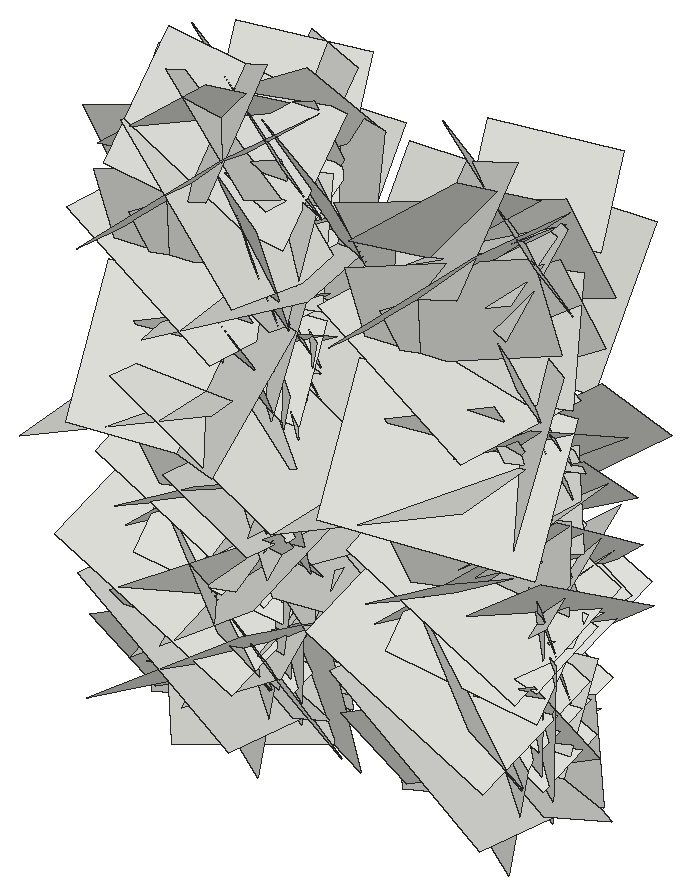
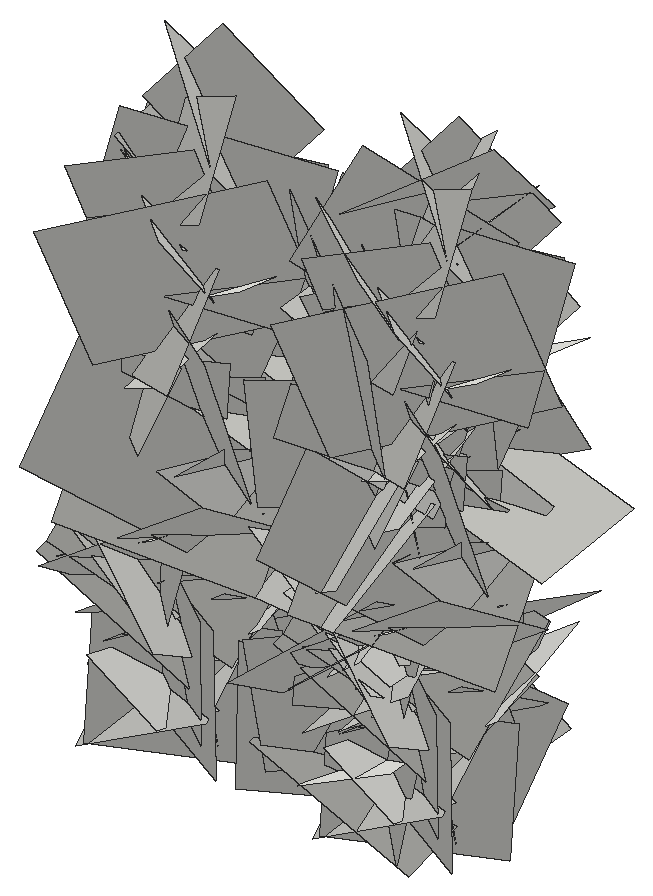
# SketchUp Ruby script. Lengths in inches.
U = 1.inch
M = Sketchup.active_model
def pt(a) = Geom::Point3d.new(a.map { |v| v * U })
def face(e, loops, mat)
  f = e.add_face(loops[0].map { |a| pt(a) })
  loops[1..].each { |l| e.add_face(l.map { |a| pt(a) }).erase! }
  f.material = f.back_material = mat if mat
  f
end
# faces: each face lists its corners as indices into pts; further lists are holes
def faces(e, pts, list, mat = nil) = list.each { |f| face(e, (f[0].is_a?(Array) ? f : [f]).map { |l| l.map { |i| pts[i] } }, mat) }
# xy, xz, yz: faces in a plane at the given z, y or x. An outline is a flat list of corners, or four numbers for a rectangle; further outlines are holes
def ring(l) = l.size == 4 ? [[l[0], l[1]], [l[2], l[1]], [l[2], l[3]], [l[0], l[3]]] : l.each_slice(2).to_a
def flat(e, list, mat, &to3) = list.each { |f| face(e, (f[0].is_a?(Array) ? f : [f]).map { |l| ring(l).map { |u, v| to3.(u, v) } }, mat) }
def xy(e, z, list, mat = nil) = flat(e, list, mat) { |x, y| [x, y, z] }
def xz(e, y, list, mat = nil) = flat(e, list, mat) { |x, z| [x, y, z] }
def yz(e, x, list, mat = nil) = flat(e, list, mat) { |y, z| [x, y, z] }
def lines(e, pts, list) = list.each { |a, b| e.add_line(pt(pts[a]), pt(pts[b])) }
# prism: a flat outline (further loops are holes) pulled along v
def prism(e, loops, v, mat = nil)
  f = face(e, loops, mat); d = Geom::Vector3d.new(v.map { |x| x * U })
  f.pushpull(f.normal.samedirection?(d) ? d.length : -d.length)
end
def box(e, o, s, mat = nil) = prism(e, [[o, [o[0] + s[0], o[1], o[2]], [o[0] + s[0], o[1] + s[1], o[2]], [o[0], o[1] + s[1], o[2]]]], [0, 0, s[2]], mat)
def at(x, y, z, deg = 0) = Geom::Transformation.translation(pt([x, y, z])) * Geom::Transformation.rotation(ORIGIN, Z_AXIS, deg.degrees)
def axes(o, x, y, z) = Geom::Transformation.new([*x, 0, *y, 0, *z, 0, *pt(o).to_a, 1])
def part(name) = M.definitions.add(name)
# library, detail: a bought-in or finely detailed component or shape, given as its bounding box
def library(name, o, s) = part(name).tap { |d| box(d.entities, o, s) }
def detail(e, o, s) = box(e.add_group.entities, o, s)
def put(e, d, t, mat = nil) = e.add_instance(d, t).tap { |i| i.material = mat if mat }
def group(e, t, mat = nil) = e.add_group.tap { |g| g.transformation = t; g.material = mat if mat }.entities
root = M.entities
c1 = part("Component\#6")
p = [[0.01,0,0],[0,3.24,4.54],[4.32,3.24,4.54],[4.33,0,0]]
faces(c1.entities,p,[[0,1,2,3]])
put(root,c1,axes([400.91,170.45,6.95],[-0.13562,-0.59571,0.16409],[0.06684,0.15411,0.60864],[0.65155,-0.13981,-0.02828]))
put(root,c1,axes([404.88,170.45,6.95],[0.13562,-0.59571,0.16409],[-0.06684,0.15411,0.60864],[-0.65155,-0.13981,-0.02828]))
put(root,c1,axes([410.71,170.45,6.95],[-0.13562,-0.59571,0.16409],[0.06684,0.15411,0.60864],[0.65155,-0.13981,-0.02828]))
put(root,c1,axes([404.88,172.51,13.7],[0.18405,-0.71312,-0.93832],[0.0125,-0.94735,0.72216],[-1.2492,-0.11455,-0.13102]))
put(root,c1,axes([400.91,172.51,13.7],[-0.18405,-0.71312,-0.93832],[-0.0125,-0.94735,0.72216],[1.2492,-0.11455,-0.13102]))
put(root,c1,axes([414.68,172.51,13.7],[0.18405,-0.71312,-0.93832],[0.0125,-0.94735,0.72216],[-1.2492,-0.11455,-0.13102]))
put(root,c1,axes([404.88,166.89,12.83],[-0.13197,1.26874,-0.04114],[-0.28106,-0.06642,-1.24587],[-1.31589,-0.11305,0.27023]))
put(root,c1,axes([400.91,166.89,12.83],[0.13197,1.26874,-0.04114],[0.28106,-0.06642,-1.24587],[1.31589,-0.11305,0.27023]))
put(root,c1,axes([414.68,166.89,12.83],[-0.13197,1.26874,-0.04114],[-0.28106,-0.06642,-1.24587],[-1.31589,-0.11305,0.27023]))
put(root,c1,axes([400.91,170.4375,18.81],[-0.19883,-0.70321,0.38228],[-0.06935,0.40479,0.71252],[0.84558,-0.13215,0.14832]))
put(root,c1,axes([404.88,170.4375,18.81],[0.19883,-0.70321,0.38228],[0.06935,0.40479,0.71252],[-0.84558,-0.13215,0.14832]))
put(root,c1,axes([410.71,170.4375,18.81],[-0.19883,-0.70321,0.38228],[-0.06935,0.40479,0.71252],[0.84558,-0.13215,0.14832]))
put(root,c1,axes([404.88,172.01,0.23],[0.18306,-1.21621,0.26629],[0.00588,0.26959,1.22768],[-1.31971,-0.16751,0.04241]))
put(root,c1,axes([400.91,172.01,0.23],[-0.18306,-1.21621,0.26629],[-0.00588,0.26959,1.22768],[1.31971,-0.16751,0.04241]))
put(root,c1,axes([414.68,172.01,0.23],[0.18306,-1.21621,0.26629],[0.00588,0.26959,1.22768],[-1.31971,-0.16751,0.04241]))
put(root,c1,axes([404.88,167.43,21.54],[-0.05686,1.16606,-0.16138],[0.18622,-0.15181,-1.15529],[-1.23383,-0.07665,-0.16693]))
put(root,c1,axes([400.91,167.43,21.54],[0.05686,1.16606,-0.16138],[-0.18622,-0.15181,-1.15529],[1.23383,-0.07665,-0.16693]))
put(root,c1,axes([414.68,167.43,21.54],[-0.05686,1.16606,-0.16138],[0.18622,-0.15181,-1.15529],[-1.23383,-0.07665,-0.16693]))
put(root,c1,axes([404.88,170.29,20.28],[-0.01759,0.35165,-0.94572],[-0.09141,-0.94289,-0.34909],[-1.06561,0.07508,0.04555]))
put(root,c1,axes([400.91,170.29,20.28],[0.01759,0.35165,-0.94572],[0.09141,-0.94289,-0.34909],[1.06561,0.07508,0.04555]))
put(root,c1,axes([414.68,170.29,20.28],[-0.01759,0.35165,-0.94572],[-0.09141,-0.94289,-0.34909],[-1.06561,0.07508,0.04555]))
put(root,c1,axes([404.88,166.61,20.4],[-0.01588,0.7114,0.79833],[0.18087,0.78977,-0.70057],[-1.11894,0.11757,-0.12458]))
put(root,c1,axes([400.91,166.61,20.4],[0.01588,0.7114,0.79833],[-0.18087,0.78977,-0.70057],[1.11894,0.11757,-0.12458]))
put(root,c1,axes([414.68,166.61,20.4],[-0.01588,0.7114,0.79833],[0.18087,0.78977,-0.70057],[-1.11894,0.11757,-0.12458]))
put(root,c1,axes([400.91,169.875,11.58],[-0.08121,-0.31714,0.54408],[0.11401,0.53345,0.32609],[0.65774,-0.13162,0.01065]))
put(root,c1,axes([404.88,169.875,11.58],[0.08121,-0.31714,0.54408],[-0.11401,0.53345,0.32609],[-0.65774,-0.13162,0.01065]))
put(root,c1,axes([410.71,169.875,11.58],[-0.08121,-0.31714,0.54408],[0.11401,0.53345,0.32609],[0.65774,-0.13162,0.01065]))
put(root,c1,axes([404.88,169.82,1.95],[0.02915,-0.64251,0.76006],[0.08177,0.75943,0.6392],[-1.05178,0.04123,0.07076]))
put(root,c1,axes([400.91,169.82,1.95],[-0.02915,-0.64251,0.76006],[-0.08177,0.75943,0.6392],[1.05178,0.04123,0.07076]))
put(root,c1,axes([414.68,169.82,1.95],[0.02915,-0.64251,0.76006],[0.08177,0.75943,0.6392],[-1.05178,0.04123,0.07076]))
put(root,c1,axes([404.88,173.1,4.27],[-0.006,-1.20261,-0.38975],[0.07836,-0.3894,1.20046],[-1.33775,-0.01742,0.07206]))
put(root,c1,axes([400.91,173.1,4.27],[0.006,-1.20261,-0.38975],[-0.07836,-0.3894,1.20046],[1.33775,-0.01742,0.07206]))
put(root,c1,axes([414.68,173.1,4.27],[-0.006,-1.20261,-0.38975],[0.07836,-0.3894,1.20046],[-1.33775,-0.01742,0.07206]))
put(root,c1,axes([400.91,169.57,7.53],[0.02893,-0.34038,0.60393],[-0.06424,0.60091,0.34142],[0.73203,0.06619,0.00609]))
put(root,c1,axes([404.88,169.57,7.53],[-0.02893,-0.34038,0.60393],[0.06424,0.60091,0.34142],[-0.73203,0.06619,0.00609]))
put(root,c1,axes([410.71,169.57,7.53],[0.02893,-0.34038,0.60393],[-0.06424,0.60091,0.34142],[0.73203,0.06619,0.00609]))
put(root,c1,axes([404.88,172.68,14.25],[-0.15371,-1.16437,-0.05617],[-0.14183,-0.0396,1.1664],[-1.22751,0.15038,-0.12774]))
put(root,c1,axes([400.91,172.68,14.25],[0.15371,-1.16437,-0.05617],[0.14183,-0.0396,1.1664],[1.22751,0.15038,-0.12774]))
put(root,c1,axes([414.68,172.68,14.25],[-0.15371,-1.16437,-0.05617],[-0.14183,-0.0396,1.1664],[-1.22751,0.15038,-0.12774]))
put(root,c1,axes([404.88,172.08,18.68],[0.05145,-0.65016,0.07549],[-0.09383,0.06848,0.64671],[-0.68743,-0.05801,-0.08262]))
put(root,c1,axes([400.91,172.08,18.68],[-0.05145,-0.65016,0.07549],[0.09383,0.06848,0.64671],[0.68743,-0.05801,-0.08262]))
put(root,c1,axes([410.71,172.08,18.68],[-0.05145,-0.65016,0.07549],[0.09383,0.06848,0.64671],[0.68743,-0.05801,-0.08262]))
put(root,c1,axes([400.91,168.08,6.15],[-0.10311,0.69666,0.5447],[-0.01855,0.54636,-0.70191],[0.9372,0.08746,0.04604]))
put(root,c1,axes([404.88,168.08,6.15],[0.10311,0.69666,0.5447],[0.01855,0.54636,-0.70191],[-0.9372,0.08746,0.04604]))
put(root,c1,axes([410.71,168.08,6.15],[-0.10311,0.69666,0.5447],[-0.01855,0.54636,-0.70191],[0.9372,0.08746,0.04604]))
put(root,c1,axes([404.88,170.37,5.28],[0.04044,0.69271,-0.86885],[-0.14808,-0.85947,-0.69137],[-1.16852,0.13289,0.05755]))
put(root,c1,axes([400.91,170.37,5.28],[-0.04044,0.69271,-0.86885],[0.14808,-0.85947,-0.69137],[1.16852,0.13289,0.05755]))
put(root,c1,axes([414.68,170.37,5.28],[0.04044,0.69271,-0.86885],[-0.14808,-0.85947,-0.69137],[-1.16852,0.13289,0.05755]))
put(root,c1,axes([404.88,171.61,19.65],[0.05512,0.44879,-0.89687],[0.12411,-0.89465,-0.44089],[-1.05579,-0.08174,-0.09865]))
put(root,c1,axes([400.91,171.61,19.65],[-0.05512,0.44879,-0.89687],[-0.12411,-0.89465,-0.44089],[1.05579,-0.08174,-0.09865]))
put(root,c1,axes([414.68,171.61,19.65],[0.05512,0.44879,-0.89687],[0.12411,-0.89465,-0.44089],[-1.05579,-0.08174,-0.09865]))
put(root,c1,axes([404.88,172.8125,18.6875],[0.10377,-0.25363,-0.96814],[-0.17625,-0.96337,0.23557],[-1.04612,0.13715,-0.13572]))
put(root,c1,axes([400.91,172.8125,18.6875],[-0.10377,-0.25363,-0.96814],[0.17625,-0.96337,0.23557],[1.04612,0.13715,-0.13572]))
put(root,c1,axes([414.68,172.8125,18.6875],[0.10377,-0.25363,-0.96814],[-0.17625,-0.96337,0.23557],[-1.04612,0.13715,-0.13572]))
put(root,c1,axes([404.88,173.43,2.26],[-0.13173,-0.86629,-0.47025],[0.00519,-0.47451,0.87284],[-1.04483,0.10686,0.06363]))
put(root,c1,axes([400.91,173.43,2.26],[0.13173,-0.86629,-0.47025],[-0.00519,-0.47451,0.87284],[1.04483,0.10686,0.06363]))
put(root,c1,axes([414.68,173.43,2.26],[-0.13173,-0.86629,-0.47025],[0.00519,-0.47451,0.87284],[-1.04483,0.10686,0.06363]))
put(root,c1,axes([400.91,172.62,2.82],[-0.11022,-0.07985,-0.84847],[0.01268,-0.85481,0.07898],[0.90326,0.00226,-0.10464]))
put(root,c1,axes([404.88,172.62,2.82],[0.11022,-0.07985,-0.84847],[-0.01268,-0.85481,0.07898],[-0.90326,0.00226,-0.10464]))
put(root,c1,axes([410.71,172.62,2.82],[-0.11022,-0.07985,-0.84847],[0.01268,-0.85481,0.07898],[0.90326,0.00226,-0.10464]))
put(root,c1,axes([404.88,172.18,10.26],[-0.13568,0.14362,-0.9313],[-0.0793,-0.93844,-0.13444],[-0.9957,0.05517,0.13761]))
put(root,c1,axes([414.68,172.18,10.26],[-0.13568,0.14362,-0.9313],[-0.0793,-0.93844,-0.13444],[-0.9957,0.05517,0.13761]))
put(root,c1,axes([400.91,172.18,10.26],[0.13568,0.14362,-0.9313],[0.0793,-0.93844,-0.13444],[0.9957,0.05517,0.13761]))
put(root,c1,axes([400.91,169.25,3.37],[-0.12984,0.58451,0.34416],[-0.01188,0.34794,-0.59491],[0.71891,0.11132,0.05233]))
put(root,c1,axes([404.88,169.25,3.37],[0.12984,0.58451,0.34416],[0.01188,0.34794,-0.59491],[-0.71891,0.11132,0.05233]))
put(root,c1,axes([410.71,169.25,3.37],[-0.12984,0.58451,0.34416],[-0.01188,0.34794,-0.59491],[0.71891,0.11132,0.05233]))
put(root,c1,axes([404.88,174.625,6.88],[-0.07025,-1.10898,-0.49527],[0.16839,-0.49966,1.09755],[-1.27636,-0.00489,0.17206]))
put(root,c1,axes([400.91,174.625,6.88],[0.07025,-1.10898,-0.49527],[-0.16839,-0.49966,1.09755],[1.27636,-0.00489,0.17206]))
put(root,c1,axes([414.68,174.625,6.88],[-0.07025,-1.10898,-0.49527],[0.16839,-0.49966,1.09755],[-1.27636,-0.00489,0.17206]))
put(root,c1,axes([404.88,173.47,4.9],[-0.07332,-0.2848,-0.87141],[0.0336,-0.87411,0.28317],[-0.9712,-0.00874,0.07558]))
put(root,c1,axes([400.91,173.47,4.9],[0.07332,-0.2848,-0.87141],[-0.0336,-0.87411,0.28317],[0.9712,-0.00874,0.07558]))
put(root,c1,axes([414.68,173.47,4.9],[-0.07332,-0.2848,-0.87141],[0.0336,-0.87411,0.28317],[-0.9712,-0.00874,0.07558]))
put(root,c1,axes([400.91,169.67,8.54],[-0.12628,0.08221,0.86907],[-0.11161,0.86937,-0.09667],[0.91857,0.11693,0.10773]))
put(root,c1,axes([404.88,169.67,8.54],[0.12628,0.08221,0.86907],[0.11161,0.86937,-0.09667],[-0.91857,0.11693,0.10773]))
put(root,c1,axes([410.71,169.67,8.54],[-0.12628,0.08221,0.86907],[-0.11161,0.86937,-0.09667],[0.91857,0.11693,0.10773]))
put(root,c1,axes([400.91,173.61,18.42],[0.00387,-0.64214,-0.38262],[0.01033,-0.38255,0.64212],[0.79227,0.00812,-0.0065]))
put(root,c1,axes([404.88,173.61,18.42],[-0.00387,-0.64214,-0.38262],[-0.01033,-0.38255,0.64212],[-0.79227,0.00812,-0.0065]))
put(root,c1,axes([410.71,173.61,18.42],[0.00387,-0.64214,-0.38262],[0.01033,-0.38255,0.64212],[0.79227,0.00812,-0.0065]))
put(root,c1,axes([404.88,173.47,6.03],[0.02519,-0.71274,-0.22366],[-0.1783,-0.22314,0.69319],[-0.7715,0.02829,-0.1675]))
put(root,c1,axes([400.91,173.47,6.03],[-0.02519,-0.71274,-0.22366],[0.1783,-0.22314,0.69319],[0.7715,0.02829,-0.1675]))
put(root,c1,axes([414.68,173.47,6.03],[0.02519,-0.71274,-0.22366],[-0.1783,-0.22314,0.69319],[-0.7715,0.02829,-0.1675]))
put(root,c1,axes([404.88,170.23,14.27],[0.02775,1.05616,-0.50439],[0.01222,-0.50473,-1.05626],[-1.24058,0.01865,-0.02169]))
put(root,c1,axes([400.91,170.23,14.27],[-0.02775,1.05616,-0.50439],[-0.01222,-0.50473,-1.05626],[1.24058,0.01865,-0.02169]))
put(root,c1,axes([414.68,170.23,14.27],[0.02775,1.05616,-0.50439],[0.01222,-0.50473,-1.05626],[-1.24058,0.01865,-0.02169]))
put(root,c1,axes([404.88,172.3,17.31],[0.17712,-0.66279,0.75583],[-0.05377,0.75967,0.67737],[-1.06423,-0.14869,0.09157]))
put(root,c1,axes([400.91,172.3,17.31],[-0.17712,-0.66279,0.75583],[0.05377,0.75967,0.67737],[1.06423,-0.14869,0.09157]))
put(root,c1,axes([414.68,172.3,17.31],[0.17712,-0.66279,0.75583],[-0.05377,0.75967,0.67737],[-1.06423,-0.14869,0.09157]))
put(root,c1,axes([404.88,171.9,21.66],[-0.05821,0.63814,-1.10333],[-0.23209,-1.09266,-0.62107],[-1.33097,0.16262,0.15656]))
put(root,c1,axes([400.91,171.9,21.66],[0.05821,0.63814,-1.10333],[0.23209,-1.09266,-0.62107],[1.33097,0.16262,0.15656]))
put(root,c1,axes([414.68,171.9,21.66],[-0.05821,0.63814,-1.10333],[-0.23209,-1.09266,-0.62107],[-1.33097,0.16262,0.15656]))
put(root,c1,axes([400.91,171.64,6.09],[-0.04085,-0.22846,0.61977],[0.06336,0.61707,0.23119],[0.6973,-0.06945,0.0153]))
put(root,c1,axes([404.88,171.64,6.09],[0.04085,-0.22846,0.61977],[-0.06336,0.61707,0.23119],[-0.6973,-0.06945,0.0153]))
put(root,c1,axes([410.71,171.64,6.09],[-0.04085,-0.22846,0.61977],[0.06336,0.61707,0.23119],[0.6973,-0.06945,0.0153]))
put(root,c1,axes([404.88,170.14,10.52],[-0.06349,0.95893,0.01002],[0.03302,0.01198,-0.96028],[-1.01599,-0.05954,-0.03183]))
put(root,c1,axes([400.91,170.14,10.52],[0.06349,0.95893,0.01002],[-0.03302,0.01198,-0.96028],[1.01599,-0.05954,-0.03183]))
put(root,c1,axes([414.68,170.14,10.52],[-0.06349,0.95893,0.01002],[0.03302,0.01198,-0.96028],[-1.01599,-0.05954,-0.03183]))
put(root,c1,axes([400.91,174.87,19.3],[-0.1513,-0.51657,-0.73784],[-0.06675,-0.7395,0.52991],[0.9524,-0.13389,-0.08008]))
put(root,c1,axes([404.88,174.87,19.3],[0.1513,-0.51657,-0.73784],[0.06675,-0.7395,0.52991],[-0.9524,-0.13389,-0.08008]))
put(root,c1,axes([410.71,174.87,19.3],[-0.1513,-0.51657,-0.73784],[-0.06675,-0.7395,0.52991],[0.9524,-0.13389,-0.08008]))
put(root,c1,axes([404.88,172.92,11.6],[-0.15777,-0.72106,0.34948],[0.01112,0.35368,0.73418],[-0.84929,0.13857,-0.05531]))
put(root,c1,axes([400.91,172.92,11.6],[0.15777,-0.72106,0.34948],[-0.01112,0.35368,0.73418],[0.84929,0.13857,-0.05531]))
put(root,c1,axes([414.68,172.92,11.6],[-0.15777,-0.72106,0.34948],[0.01112,0.35368,0.73418],[-0.84929,0.13857,-0.05531]))
put(root,c1,axes([404.88,169.35,10.4],[0.15861,0.37048,1.309],[-0.06067,1.31744,-0.36632],[-1.44077,-0.01469,0.15953]))
put(root,c1,axes([400.91,169.35,10.4],[-0.15861,0.37048,1.309],[0.06067,1.31744,-0.36632],[1.44077,-0.01469,0.15953]))
put(root,c1,axes([414.68,169.35,10.4],[0.15861,0.37048,1.309],[-0.06067,1.31744,-0.36632],[-1.44077,-0.01469,0.15953]))
put(root,c1,axes([404.88,171.5,10.51],[-0.09816,1.08592,-0.68794],[0.27584,-0.65961,-1.07622],[-1.33441,-0.21623,-0.17187]))
put(root,c1,axes([400.91,171.5,10.51],[0.09816,1.08592,-0.68794],[-0.27584,-0.65961,-1.07622],[1.33441,-0.21623,-0.17187]))
put(root,c1,axes([414.68,171.5,10.51],[-0.09816,1.08592,-0.68794],[0.27584,-0.65961,-1.07622],[-1.33441,-0.21623,-0.17187]))
put(root,c1,axes([404.88,170.67,8.7],[0.18467,1.04701,-0.56036],[0.0341,-0.57031,-1.0556],[-1.25832,0.1382,-0.11085]))
put(root,c1,axes([400.91,170.67,8.7],[-0.18467,1.04701,-0.56036],[-0.0341,-0.57031,-1.0556],[1.25832,0.1382,-0.11085]))
put(root,c1,axes([414.68,170.67,8.7],[0.18467,1.04701,-0.56036],[0.0341,-0.57031,-1.0556],[-1.25832,0.1382,-0.11085]))
put(root,c1,axes([404.88,174.22,3.89],[-0.08779,-0.72671,-0.31501],[-0.02258,-0.31457,0.73129],[-0.83927,0.08448,0.01327]))
put(root,c1,axes([400.91,174.22,3.89],[0.08779,-0.72671,-0.31501],[0.02258,-0.31457,0.73129],[0.83927,0.08448,0.01327]))
put(root,c1,axes([414.68,174.22,3.89],[-0.08779,-0.72671,-0.31501],[-0.02258,-0.31457,0.73129],[-0.83927,0.08448,0.01327]))
put(root,c1,axes([404.88,174.19,-1.125],[0.19779,-1.01545,0.55728],[-0.13113,0.54376,1.03224],[-1.22079,-0.22293,-0.02059]))
put(root,c1,axes([400.91,174.19,-1.125],[-0.19779,-1.01545,0.55728],[0.13113,0.54376,1.03224],[1.22079,-0.22293,-0.02059]))
put(root,c1,axes([414.68,174.19,-1.125],[0.19779,-1.01545,0.55728],[-0.13113,0.54376,1.03224],[-1.22079,-0.22293,-0.02059]))
put(root,c1,axes([400.91,171.41,10.85],[-0.07762,0.04197,0.59758],[0.0194,0.6019,-0.04003],[0.6347,-0.01326,0.07431]))
put(root,c1,axes([404.88,171.41,10.85],[0.07762,0.04197,0.59758],[-0.0194,0.6019,-0.04003],[-0.6347,-0.01326,0.07431]))
put(root,c1,axes([410.71,171.41,10.85],[-0.07762,0.04197,0.59758],[0.0194,0.6019,-0.04003],[0.6347,-0.01326,0.07431]))
put(root,c1,axes([404.88,173.32,3.72],[-0.0912,0.22313,-1.04907],[-0.17676,-1.04242,-0.20804],[-1.12306,0.14594,0.11794]))
put(root,c1,axes([400.91,173.32,3.72],[0.0912,0.22313,-1.04907],[0.17676,-1.04242,-0.20804],[1.12306,0.14594,0.11794]))
put(root,c1,axes([414.68,173.32,3.72],[-0.0912,0.22313,-1.04907],[-0.17676,-1.04242,-0.20804],[-1.12306,0.14594,0.11794]))
put(root,c1,axes([400.91,173.27,2.31],[0.02745,-0.60704,0.2793],[-0.09658,0.2737,0.6033],[0.70169,0.06142,0.07211]))
put(root,c1,axes([404.88,173.27,2.31],[-0.02745,-0.60704,0.2793],[0.09658,0.2737,0.6033],[-0.70169,0.06142,0.07211]))
put(root,c1,axes([410.71,173.27,2.31],[0.02745,-0.60704,0.2793],[-0.09658,0.2737,0.6033],[0.70169,0.06142,0.07211]))
put(root,c1,axes([404.88,172.23,12.17],[-0.04321,-0.56467,0.8488],[0.06772,0.84639,0.56613],[-1.07851,0.07577,0.00154]))
put(root,c1,axes([400.91,172.23,12.17],[0.04321,-0.56467,0.8488],[-0.06772,0.84639,0.56613],[1.07851,0.07577,0.00154]))
put(root,c1,axes([414.68,172.23,12.17],[-0.04321,-0.56467,0.8488],[0.06772,0.84639,0.56613],[-1.07851,0.07577,0.00154]))
put(root,c1,axes([404.88,170.77,1.94],[-0.10305,0.14958,1.1623],[0.03,1.16625,-0.14772],[-1.24184,0.01576,-0.10002]))
put(root,c1,axes([400.91,170.77,1.94],[0.10305,0.14958,1.1623],[-0.03,1.16625,-0.14772],[1.24184,0.01576,-0.10002]))
put(root,c1,axes([414.68,170.77,1.94],[-0.10305,0.14958,1.1623],[0.03,1.16625,-0.14772],[-1.24184,0.01576,-0.10002]))
put(root,c1,axes([404.88,172.28,10.96],[-0.19399,-0.26613,0.68464],[0.06344,0.69782,0.28725],[-0.77602,0.12358,-0.14766]))
put(root,c1,axes([400.91,172.28,10.96],[0.19399,-0.26613,0.68464],[-0.06344,0.69782,0.28725],[0.77602,0.12358,-0.14766]))
put(root,c1,axes([414.68,172.28,10.96],[-0.19399,-0.26613,0.68464],[0.06344,0.69782,0.28725],[-0.77602,0.12358,-0.14766]))
put(root,c1,axes([404.88,172.17,3.88],[-0.10658,-0.21665,0.83392],[0.00523,0.83942,0.21867],[-0.91328,0.03009,-0.09606]))
put(root,c1,axes([400.91,172.17,3.88],[0.10658,-0.21665,0.83392],[-0.00523,0.83942,0.21867],[0.91328,0.03009,-0.09606]))
put(root,c1,axes([414.68,172.17,3.88],[-0.10658,-0.21665,0.83392],[0.00523,0.83942,0.21867],[-0.91328,0.03009,-0.09606]))
put(root,c1,axes([404.88,172.79,12.08],[-0.24348,0.91998,-0.78066],[-0.03668,-0.79938,-0.93185],[-1.27843,-0.15228,0.17542]))
put(root,c1,axes([400.91,172.79,12.08],[0.24348,0.91998,-0.78066],[0.03668,-0.79938,-0.93185],[1.27843,-0.15228,0.17542]))
put(root,c1,axes([414.68,172.79,12.08],[-0.24348,0.91998,-0.78066],[-0.03668,-0.79938,-0.93185],[-1.27843,-0.15228,0.17542]))
put(root,c1,axes([404.88,171.28,0.09],[0.0277,-0.00252,1.28462],[-0.09278,1.2819,0.0043],[-1.35854,-0.08759,0.0259]))
put(root,c1,axes([414.68,171.28,0.09],[0.0277,-0.00252,1.28462],[-0.09278,1.2819,0.0043],[-1.35854,-0.08759,0.0259]))
put(root,c1,axes([400.91,171.28,0.09],[-0.0277,-0.00252,1.28462],[0.09278,1.2819,0.0043],[1.35854,-0.08759,0.0259]))
put(root,c1,axes([400.91,174.97,1.18],[-0.10067,-0.62121,-0.06126],[0.13552,-0.08001,0.61313],[0.64765,-0.07982,-0.13782]))
put(root,c1,axes([404.88,174.97,1.18],[0.10067,-0.62121,-0.06126],[-0.13552,-0.08001,0.61313],[-0.64765,-0.07982,-0.13782]))
put(root,c1,axes([410.71,174.97,1.18],[-0.10067,-0.62121,-0.06126],[0.13552,-0.08001,0.61313],[0.64765,-0.07982,-0.13782]))
put(root,c1,axes([404.88,176.36,18.92],[-0.19548,-0.4632,-1.27504],[0.04093,-1.28804,0.46234],[-1.43738,0.02631,0.18657]))
put(root,c1,axes([400.91,176.36,18.92],[0.19548,-0.4632,-1.27504],[-0.04093,-1.28804,0.46234],[1.43738,0.02631,0.18657]))
put(root,c1,axes([414.68,176.36,18.92],[-0.19548,-0.4632,-1.27504],[0.04093,-1.28804,0.46234],[-1.43738,0.02631,0.18657]))
put(root,c1,axes([404.88,176.11,6.43],[-0.23133,-1.0261,-0.61864],[-0.04368,-0.62202,1.04624],[-1.2693,0.20842,0.07674]))
put(root,c1,axes([400.91,176.11,6.43],[0.23133,-1.0261,-0.61864],[0.04368,-0.62202,1.04624],[1.2693,0.20842,0.07674]))
put(root,c1,axes([414.68,176.11,6.43],[-0.23133,-1.0261,-0.61864],[-0.04368,-0.62202,1.04624],[-1.2693,0.20842,0.07674]))
put(root,c1,axes([404.88,175.17,6.35],[-0.11089,-0.78923,-0.08985],[-0.10937,-0.07636,0.79084],[-0.83485,0.11483,-0.09167]))
put(root,c1,axes([400.91,175.17,6.35],[0.11089,-0.78923,-0.08985],[0.10937,-0.07636,0.79084],[0.83485,0.11483,-0.09167]))
put(root,c1,axes([414.68,175.17,6.35],[-0.11089,-0.78923,-0.08985],[-0.10937,-0.07636,0.79084],[-0.83485,0.11483,-0.09167]))
put(root,c1,axes([400.91,175.4,4.97],[0.01432,-0.74639,-0.04739],[-0.08616,-0.04858,0.74199],[0.78807,0.00825,0.08199]))
put(root,c1,axes([404.88,175.4,4.97],[-0.01432,-0.74639,-0.04739],[0.08616,-0.04858,0.74199],[-0.78807,0.00825,0.08199]))
put(root,c1,axes([410.71,175.4,4.97],[0.01432,-0.74639,-0.04739],[-0.08616,-0.04858,0.74199],[0.78807,0.00825,0.08199]))
put(root,c1,axes([404.88,173.68,14.42],[-0.07839,0.88361,-0.83437],[0.27617,-0.80495,-0.87555],[-1.25826,-0.23172,-0.14019]))
put(root,c1,axes([400.91,173.68,14.42],[0.07839,0.88361,-0.83437],[-0.27617,-0.80495,-0.87555],[1.25826,-0.23172,-0.14019]))
put(root,c1,axes([414.68,173.68,14.42],[-0.07839,0.88361,-0.83437],[0.27617,-0.80495,-0.87555],[-1.25826,-0.23172,-0.14019]))
put(root,c1,axes([400.91,171.94,19.49],[-0.08782,0.36838,0.63269],[0.00702,0.63708,-0.37006],[0.77601,0.03592,0.07495]))
put(root,c1,axes([404.88,171.94,19.49],[0.08782,0.36838,0.63269],[-0.00702,0.63708,-0.37006],[-0.77601,0.03592,0.07495]))
put(root,c1,axes([410.71,171.94,19.49],[-0.08782,0.36838,0.63269],[0.00702,0.63708,-0.37006],[0.77601,0.03592,0.07495]))
put(root,c1,axes([404.88,170.9375,7.01],[-0.11124,0.9843,0.53665],[0.15751,0.54645,-0.97322],[-1.17787,-0.01989,-0.18083]))
put(root,c1,axes([400.91,170.9375,7.01],[0.11124,0.9843,0.53665],[-0.15751,0.54645,-0.97322],[1.17787,-0.01989,-0.18083]))
put(root,c1,axes([414.68,170.9375,7.01],[-0.11124,0.9843,0.53665],[0.15751,0.54645,-0.97322],[-1.17787,-0.01989,-0.18083]))
